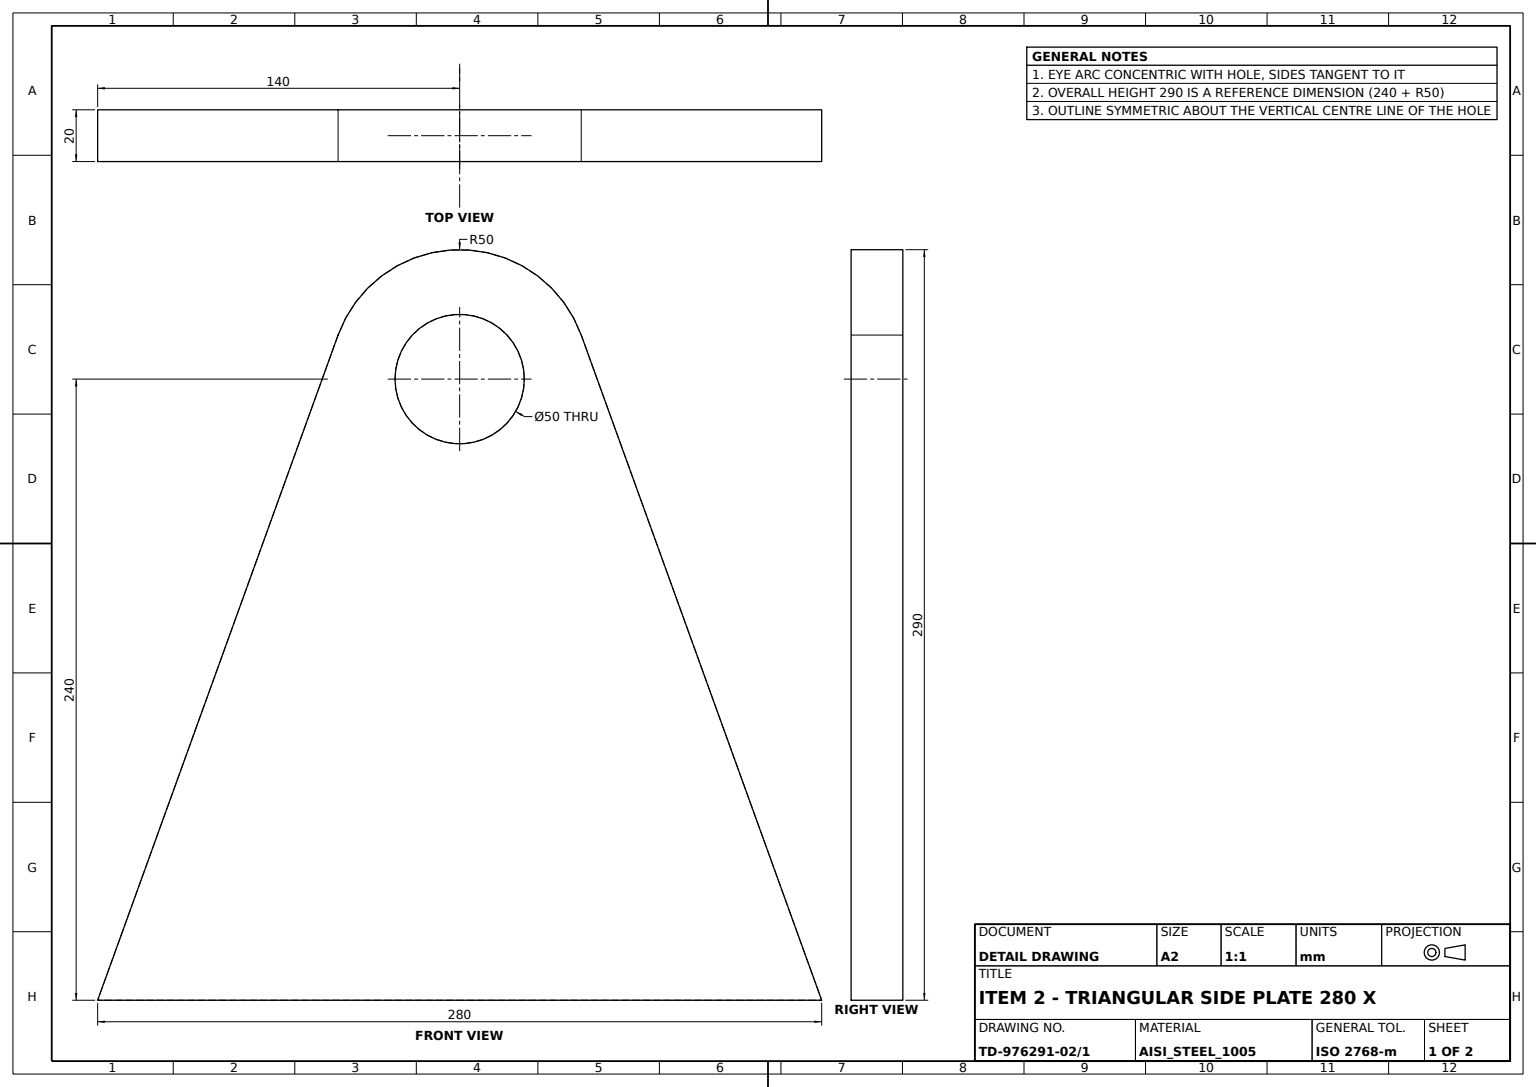
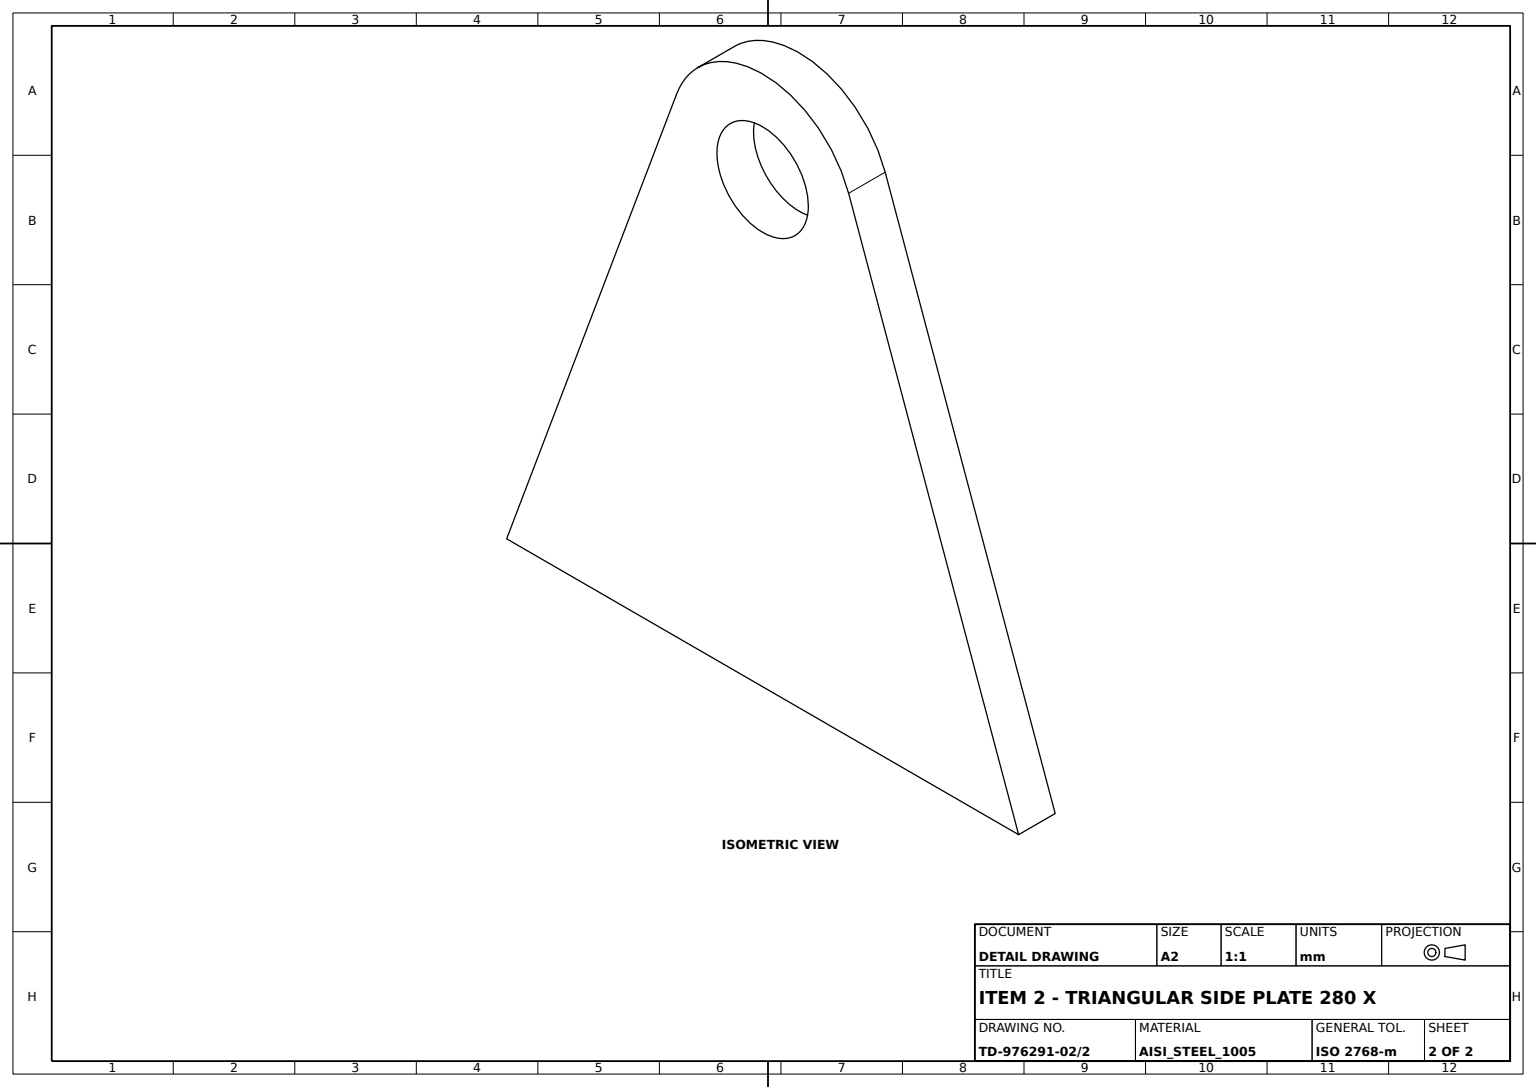
ISO-10303-21;
HEADER;
FILE_DESCRIPTION((''),'2;1');
FILE_NAME('','',(''),(''),'','','');
FILE_SCHEMA(('AUTOMOTIVE_DESIGN'));
ENDSEC;
DATA;
#1=APPLICATION_CONTEXT('');
#2=PRODUCT_CONTEXT('',#1,'mechanical');
#3=PRODUCT('','','',(#2));
#4=PRODUCT_DEFINITION_FORMATION('','',#3);
#5=PRODUCT_DEFINITION_CONTEXT('',#1,'design');
#6=PRODUCT_DEFINITION('','',#4,#5);
#7=PRODUCT_DEFINITION_SHAPE('','',#6);
#8=(LENGTH_UNIT()NAMED_UNIT(*)SI_UNIT(.MILLI.,.METRE.));
#9=(NAMED_UNIT(*)PLANE_ANGLE_UNIT()SI_UNIT($,.RADIAN.));
#10=(NAMED_UNIT(*)SI_UNIT($,.STERADIAN.)SOLID_ANGLE_UNIT());
#11=UNCERTAINTY_MEASURE_WITH_UNIT(LENGTH_MEASURE(0.005),#8,'distance_accuracy_value','');
#12=(GEOMETRIC_REPRESENTATION_CONTEXT(3)GLOBAL_UNCERTAINTY_ASSIGNED_CONTEXT((#11))GLOBAL_UNIT_ASSIGNED_CONTEXT((#8,#9,#10))REPRESENTATION_CONTEXT('',''));
#13=CARTESIAN_POINT('',(140.,-20.,0.));
#14=VERTEX_POINT('',#13);
#15=CARTESIAN_POINT('',(47.017566,-20.,257.010247));
#16=VERTEX_POINT('',#15);
#17=DIRECTION('',(-0.340204936,0.,0.940351318));
#18=VECTOR('',#17,1000.);
#19=LINE('',#13,#18);
#20=EDGE_CURVE('',#14,#16,#19,.T.);
#21=ORIENTED_EDGE('',*,*,#20,.F.);
#22=CARTESIAN_POINT('',(140.,0.,0.));
#23=VERTEX_POINT('',#22);
#24=DIRECTION('',(0.,1.,0.));
#25=VECTOR('',#24,1000.);
#26=LINE('',#13,#25);
#27=EDGE_CURVE('',#14,#23,#26,.T.);
#28=ORIENTED_EDGE('',*,*,#27,.T.);
#29=CARTESIAN_POINT('',(47.017566,0.,257.010247));
#30=VERTEX_POINT('',#29);
#31=LINE('',#22,#18);
#32=EDGE_CURVE('',#23,#30,#31,.T.);
#33=ORIENTED_EDGE('',*,*,#32,.T.);
#34=LINE('',#15,#25);
#35=EDGE_CURVE('',#16,#30,#34,.T.);
#36=ORIENTED_EDGE('',*,*,#35,.F.);
#37=EDGE_LOOP('',(#21,#28,#33,#36));
#38=FACE_BOUND('',#37,.T.);
#39=DIRECTION('',(-0.940351318,0.,-0.340204936));
#40=AXIS2_PLACEMENT_3D('',#13,#39,#17);
#41=PLANE('',#40);
#42=ADVANCED_FACE('',(#38),#41,.F.);
#43=CARTESIAN_POINT('',(-140.,-20.,0.));
#44=VERTEX_POINT('',#43);
#45=DIRECTION('',(1.,0.,0.));
#46=VECTOR('',#45,1000.);
#47=LINE('',#43,#46);
#48=EDGE_CURVE('',#44,#14,#47,.T.);
#49=ORIENTED_EDGE('',*,*,#48,.F.);
#50=CARTESIAN_POINT('',(-140.,0.,0.));
#51=VERTEX_POINT('',#50);
#52=LINE('',#43,#25);
#53=EDGE_CURVE('',#44,#51,#52,.T.);
#54=ORIENTED_EDGE('',*,*,#53,.T.);
#55=LINE('',#50,#46);
#56=EDGE_CURVE('',#51,#23,#55,.T.);
#57=ORIENTED_EDGE('',*,*,#56,.T.);
#58=ORIENTED_EDGE('',*,*,#27,.F.);
#59=EDGE_LOOP('',(#49,#54,#57,#58));
#60=FACE_BOUND('',#59,.T.);
#61=DIRECTION('',(0.,0.,1.));
#62=AXIS2_PLACEMENT_3D('',#43,#61,#45);
#63=PLANE('',#62);
#64=ADVANCED_FACE('',(#60),#63,.F.);
#65=CARTESIAN_POINT('',(25.,-20.,240.));
#66=VERTEX_POINT('',#65);
#67=CARTESIAN_POINT('',(0.,-20.,240.));
#68=DIRECTION('',(0.,-1.,0.));
#69=AXIS2_PLACEMENT_3D('',#67,#68,#45);
#70=CIRCLE('',#69,25.);
#71=EDGE_CURVE('',#66,#66,#70,.T.);
#72=ORIENTED_EDGE('',*,*,#71,.T.);
#73=EDGE_LOOP('',(#72));
#74=FACE_BOUND('',#73,.T.);
#75=CARTESIAN_POINT('',(25.,0.,240.));
#76=VERTEX_POINT('',#75);
#77=CARTESIAN_POINT('',(0.,0.,240.));
#78=AXIS2_PLACEMENT_3D('',#77,#68,#45);
#79=CIRCLE('',#78,25.);
#80=EDGE_CURVE('',#76,#76,#79,.T.);
#81=ORIENTED_EDGE('',*,*,#80,.F.);
#82=EDGE_LOOP('',(#81));
#83=FACE_BOUND('',#82,.T.);
#84=AXIS2_PLACEMENT_3D('',#67,#24,#61);
#85=CYLINDRICAL_SURFACE('',#84,25.);
#86=ADVANCED_FACE('',(#74,#83),#85,.F.);
#87=ORIENTED_EDGE('',*,*,#35,.T.);
#88=CARTESIAN_POINT('',(-47.017566,0.,257.010247));
#89=VERTEX_POINT('',#88);
#90=CIRCLE('',#78,50.);
#91=EDGE_CURVE('',#30,#89,#90,.T.);
#92=ORIENTED_EDGE('',*,*,#91,.T.);
#93=CARTESIAN_POINT('',(-47.017566,-20.,257.010247));
#94=VERTEX_POINT('',#93);
#95=LINE('',#93,#25);
#96=EDGE_CURVE('',#94,#89,#95,.T.);
#97=ORIENTED_EDGE('',*,*,#96,.F.);
#98=CIRCLE('',#69,50.);
#99=EDGE_CURVE('',#16,#94,#98,.T.);
#100=ORIENTED_EDGE('',*,*,#99,.F.);
#101=EDGE_LOOP('',(#87,#92,#97,#100));
#102=FACE_BOUND('',#101,.T.);
#103=CYLINDRICAL_SURFACE('',#84,50.);
#104=ADVANCED_FACE('',(#102),#103,.T.);
#105=ORIENTED_EDGE('',*,*,#80,.T.);
#106=EDGE_LOOP('',(#105));
#107=FACE_BOUND('',#106,.T.);
#108=ORIENTED_EDGE('',*,*,#91,.F.);
#109=ORIENTED_EDGE('',*,*,#32,.F.);
#110=ORIENTED_EDGE('',*,*,#56,.F.);
#111=DIRECTION('',(-0.340204936,0.,-0.940351318));
#112=VECTOR('',#111,1000.);
#113=LINE('',#88,#112);
#114=EDGE_CURVE('',#89,#51,#113,.T.);
#115=ORIENTED_EDGE('',*,*,#114,.F.);
#116=EDGE_LOOP('',(#108,#109,#110,#115));
#117=FACE_BOUND('',#116,.T.);
#118=DIRECTION('',(0.,0.,-1.));
#119=AXIS2_PLACEMENT_3D('',#77,#68,#118);
#120=PLANE('',#119);
#121=ADVANCED_FACE('',(#107,#117),#120,.F.);
#122=ORIENTED_EDGE('',*,*,#71,.F.);
#123=EDGE_LOOP('',(#122));
#124=FACE_BOUND('',#123,.T.);
#125=ORIENTED_EDGE('',*,*,#48,.T.);
#126=ORIENTED_EDGE('',*,*,#20,.T.);
#127=ORIENTED_EDGE('',*,*,#99,.T.);
#128=LINE('',#93,#112);
#129=EDGE_CURVE('',#94,#44,#128,.T.);
#130=ORIENTED_EDGE('',*,*,#129,.T.);
#131=EDGE_LOOP('',(#125,#126,#127,#130));
#132=FACE_BOUND('',#131,.T.);
#133=AXIS2_PLACEMENT_3D('',#67,#68,#118);
#134=PLANE('',#133);
#135=ADVANCED_FACE('',(#124,#132),#134,.T.);
#136=ORIENTED_EDGE('',*,*,#129,.F.);
#137=ORIENTED_EDGE('',*,*,#96,.T.);
#138=ORIENTED_EDGE('',*,*,#114,.T.);
#139=ORIENTED_EDGE('',*,*,#53,.F.);
#140=EDGE_LOOP('',(#136,#137,#138,#139));
#141=FACE_BOUND('',#140,.T.);
#142=DIRECTION('',(0.940351318,0.,-0.340204936));
#143=AXIS2_PLACEMENT_3D('',#93,#142,#111);
#144=PLANE('',#143);
#145=ADVANCED_FACE('',(#141),#144,.F.);
#146=CLOSED_SHELL('',(#42,#64,#86,#104,#121,#135,#145));
#147=MANIFOLD_SOLID_BREP('',#146);
#148=ADVANCED_BREP_SHAPE_REPRESENTATION('',(#147),#12);
#149=SHAPE_DEFINITION_REPRESENTATION(#7,#148);
ENDSEC;
END-ISO-10303-21;
